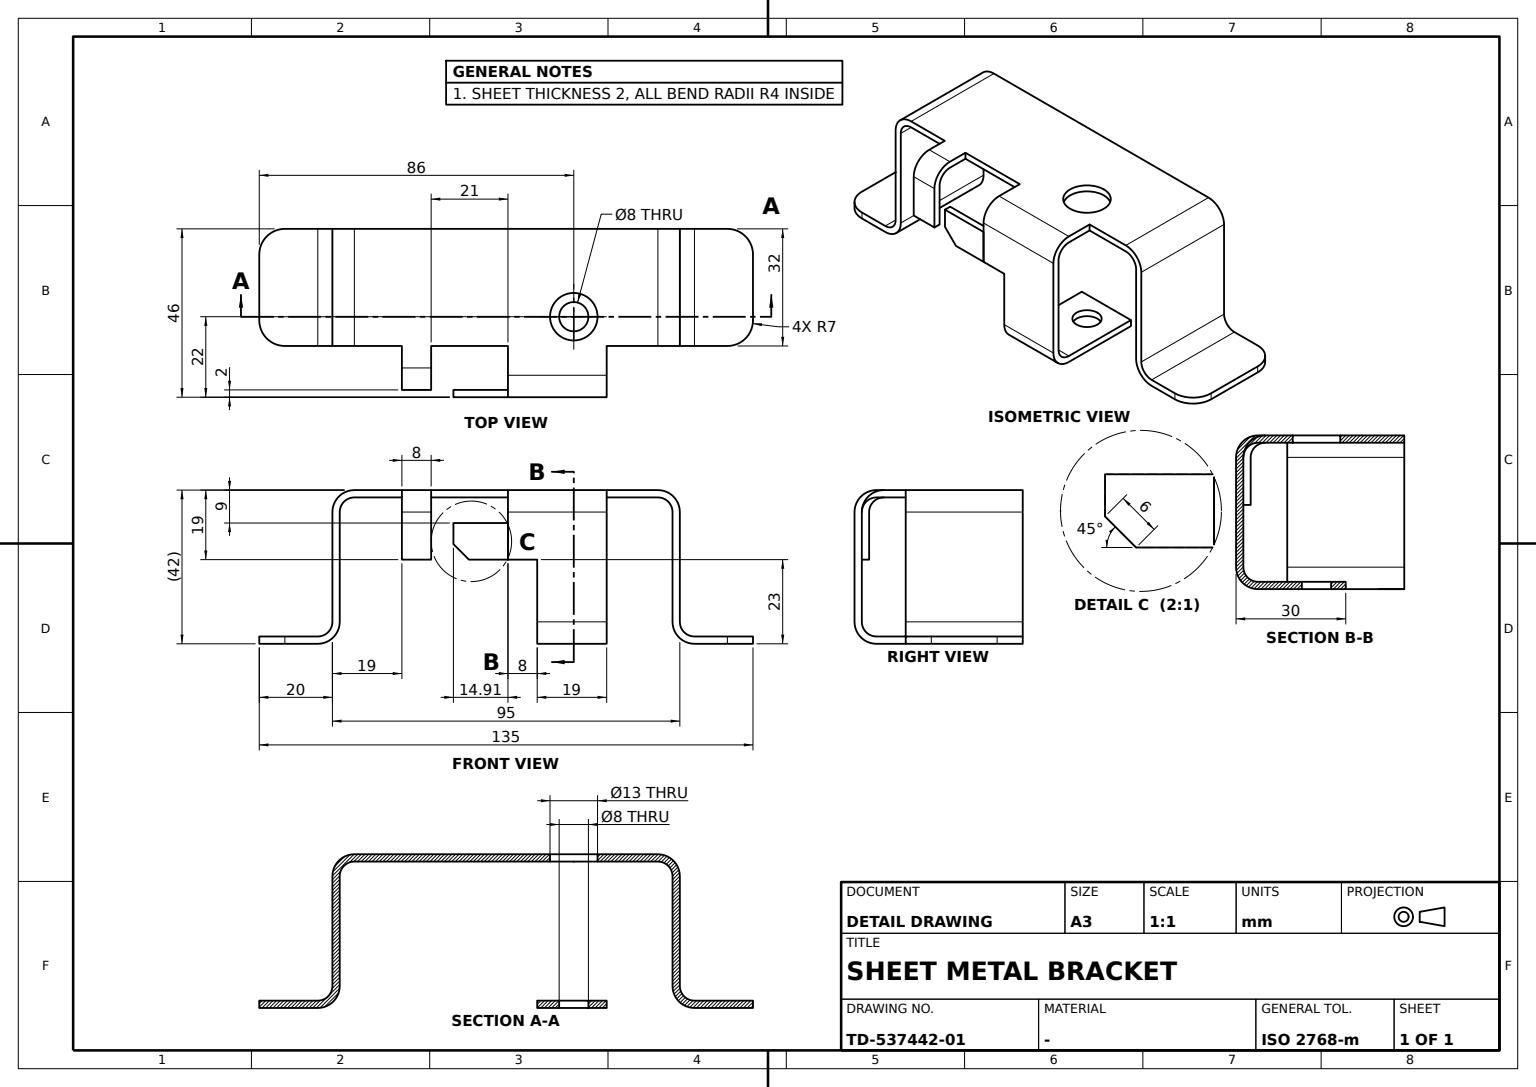
solid
v1 (0,27.5,-42)
v2 (0,27.5,-40)
e1 v1 v2 LINE
v3 (24,27.5,-40)
e2 v2 v3 LINE
v4 (28,27.5,-36)
e3 v3 v4 CIRCLE(AX(P(24,27.5,-36),D(0,1,0),D(0,0,1)),4) rev
v5 (28,27.5,-6)
e4 v5 v4 LINE
v6 (24,27.5,-2)
e5 v6 v5 CIRCLE(AX(P(24,27.5,-6),D(0,1,0),D(0,0,1)),4)
v7 (16,27.5,-2)
e6 v7 v6 LINE
v8 (16,27.5,0)
e7 v8 v7 LINE
v9 (24,27.5,0)
e8 v8 v9 LINE
v10 (30,27.5,-6)
e9 v9 v10 CIRCLE(AX(P(24,27.5,-6),D(0,1,0),D(0,0,1)),6)
v11 (30,27.5,-36)
e10 v11 v10 LINE
v12 (24,27.5,-42)
e11 v12 v11 CIRCLE(AX(P(24,27.5,-36),D(0,1,0),D(0,0,1)),6) rev
e12 v1 v12 LINE
face PLANE(AX(P(12,27.5,-42),D(0,1,0),D(1,0,0))) [e1 e2 e3 -e4 -e5 -e6 -e7 e8 e9 -e10 -e11 -e12]
v13 (24,0.5,-2)
e13 v6 v13 LINE
v14 (16,0.5,-2)
e14 v14 v13 LINE
v15 (16,-20.5,-2)
e15 v14 v15 LINE
v16 (22,-20.5,-2)
e16 v15 v16 LINE
v17 (22,-28.5,-2)
e17 v17 v16 LINE
v18 (16,-28.5,-2)
e18 v18 v17 LINE
v19 (16,-41.5,-2)
e19 v18 v19 LINE
v20 (-16,-41.5,-2)
e20 v19 v20 LINE
v21 (-16,41.5,-2)
e21 v20 v21 LINE
v22 (16,41.5,-2)
e22 v21 v22 LINE
e23 v22 v7 LINE
v23 (1.5,18.5,-2)
e24 v23 v23 CIRCLE(AX(P(8,18.5,-2),D(0,0,-1),D(-1,0,0)),6.5)
face PLANE(AX(P(16,0.5,-2),D(0,0,-1),D(0,1,0))) [e13 -e14 e15 e16 -e17 -e18 e19 e20 e21 e22 e23 e6] [-e24]
v24 (30,0.5,-6)
e25 v10 v24 LINE
v25 (30,0.5,-19)
e26 v25 v24 LINE
v26 (30,8.5,-19)
e27 v26 v25 LINE
v27 (30,8.5,-36)
e28 v26 v27 LINE
e29 v11 v27 LINE
face PLANE(AX(P(30,10.5,-2),D(1,0,0),D(0,-1,0))) [e25 -e26 -e27 e28 -e29 e10]
v28 (0,8.5,-42)
v29 (0,8.5,-40)
e30 v28 v29 LINE
e31 v29 v2 LINE
e32 v28 v1 LINE
face PLANE(AX(P(0,18,-42),D(1,0,0),D(0,0,1))) rev [e30 e31 -e1 -e32]
v30 (16,51.5,-40)
v31 (16,60.5,-40)
e33 v30 v31 LINE
v32 (16,47.5,-36)
e34 v30 v32 CIRCLE(AX(P(16,51.5,-36),D(-1,0,0),D(0,0,1)),4)
v33 (16,47.5,-6)
e35 v32 v33 LINE
v34 (16,41.5,0)
e36 v33 v34 CIRCLE(AX(P(16,41.5,-6),D(-1,0,0),D(0,0,1)),6) rev
e37 v34 v8 LINE
v35 (16,45.5,-6)
e38 v35 v22 CIRCLE(AX(P(16,41.5,-6),D(-1,0,0),D(0,0,1)),4) rev
v36 (16,45.5,-36)
e39 v35 v36 LINE
v37 (16,51.5,-42)
e40 v37 v36 CIRCLE(AX(P(16,51.5,-36),D(-1,0,0),D(0,0,1)),6)
v38 (16,60.5,-42)
e41 v37 v38 LINE
e42 v31 v38 LINE
face PLANE(AX(P(16,-47.5,0),D(-1,0,0),D(0,1,0))) rev [-e33 e34 e35 e36 e37 e7 -e23 -e38 e39 -e40 e41 -e42]
v39 (16,-47.5,-6)
v40 (16,-41.5,0)
e43 v39 v40 CIRCLE(AX(P(16,-41.5,-6),D(-1,0,0),D(0,0,1)),6)
v41 (-16,-41.5,0)
e44 v40 v41 LINE
v42 (-16,-47.5,-6)
e45 v42 v41 CIRCLE(AX(P(-16,-41.5,-6),D(-1,0,0),D(0,0,1)),6)
e46 v39 v42 LINE
face CYL(AX(P(0,-41.5,-6),D(-1,0,0),D(0,0,1)),6) [e43 e44 -e45 -e46]
v43 (-16,60.5,-42)
v44 (-9,67.5,-42)
e47 v43 v44 CIRCLE(AX(P(-9,60.5,-42),D(0,0,-1),D(-1,0,0)),7)
v45 (-16,60.5,-40)
e48 v45 v43 LINE
v46 (-9,67.5,-40)
e49 v45 v46 CIRCLE(AX(P(-9,60.5,-40),D(0,0,-1),D(-1,0,0)),7)
e50 v46 v44 LINE
face CYL(AX(P(-9,60.5,-40),D(0,0,-1),D(-1,0,0)),7) [-e47 -e48 e49 e50]
v47 (9,67.5,-40)
e51 v46 v47 LINE
v48 (-16,51.5,-40)
e52 v45 v48 LINE
e53 v30 v48 LINE
e54 v47 v31 CIRCLE(AX(P(9,60.5,-40),D(0,0,-1),D(-1,0,0)),7)
face PLANE(AX(P(28,18,-40),D(0,0,-1),D(0,-1,0))) rev [-e51 -e49 e52 -e53 e33 -e54]
v49 (-16,41.5,0)
e55 v41 v49 LINE
v50 (-16,47.5,-6)
e56 v50 v49 CIRCLE(AX(P(-16,41.5,-6),D(-1,0,0),D(0,0,1)),6) rev
v51 (-16,47.5,-36)
e57 v51 v50 LINE
e58 v48 v51 CIRCLE(AX(P(-16,51.5,-36),D(-1,0,0),D(0,0,1)),4)
v52 (-16,51.5,-42)
e59 v43 v52 LINE
v53 (-16,45.5,-36)
e60 v52 v53 CIRCLE(AX(P(-16,51.5,-36),D(-1,0,0),D(0,0,1)),6)
v54 (-16,45.5,-6)
e61 v54 v53 LINE
e62 v54 v21 CIRCLE(AX(P(-16,41.5,-6),D(-1,0,0),D(0,0,1)),4) rev
v55 (-16,-45.5,-6)
e63 v55 v20 CIRCLE(AX(P(-16,-41.5,-6),D(-1,0,0),D(0,0,1)),4)
v56 (-16,-45.5,-36)
e64 v55 v56 LINE
v57 (-16,-51.5,-42)
e65 v57 v56 CIRCLE(AX(P(-16,-51.5,-36),D(-1,0,0),D(0,0,1)),6) rev
v58 (-16,-60.5,-42)
e66 v57 v58 LINE
v59 (-16,-60.5,-40)
e67 v59 v58 LINE
v60 (-16,-51.5,-40)
e68 v60 v59 LINE
v61 (-16,-47.5,-36)
e69 v60 v61 CIRCLE(AX(P(-16,-51.5,-36),D(-1,0,0),D(0,0,1)),4) rev
e70 v61 v42 LINE
face PLANE(AX(P(-16,-59.5,-42),D(-1,0,0),D(0,1,0))) [e45 e55 -e56 -e57 -e58 -e52 e48 e59 e60 -e61 e62 -e21 -e63 e64 -e65 e66 -e67 -e68 e69 e70]
v62 (16,-45.5,-6)
e71 v62 v55 LINE
e72 v62 v19 CIRCLE(AX(P(16,-41.5,-6),D(-1,0,0),D(0,0,1)),4)
face CYL(AX(P(0,-41.5,-6),D(-1,0,0),D(0,0,1)),4) rev [e71 e63 -e20 -e72]
v63 (24,8.5,-42)
e73 v63 v27 CIRCLE(AX(P(24,8.5,-36),D(0,1,0),D(0,0,1)),6) rev
e74 v12 v63 LINE
face CYL(AX(P(24,14,-36),D(0,-1,0),D(1,0,0)),6) [e11 e29 -e73 -e74]
v64 (26,-28.5,-6)
v65 (26,-28.5,-19)
e75 v64 v65 LINE
v66 (26,-20.5,-6)
e76 v64 v66 LINE
v67 (26,-20.5,-19)
e77 v67 v66 LINE
e78 v65 v67 LINE
face PLANE(AX(P(26,0,-2),D(1,0,0),D(0,-1,0))) rev [-e75 e76 -e77 -e78]
v68 (16,-47.5,-36)
e79 v61 v68 LINE
e80 v68 v39 LINE
face PLANE(AX(P(0,-47.5,-2),D(0,-1,0),D(-1,0,0))) [e79 e80 e46 -e70]
v69 (4,18.5,-42)
e81 v69 v69 CIRCLE(AX(P(8,18.5,-42),D(0,0,-1),D(-1,0,0)),4)
v70 (4,18.5,-40)
e82 v70 v70 CIRCLE(AX(P(8,18.5,-40),D(0,0,-1),D(-1,0,0)),4)
face CYL(AX(P(8,18.5,-41),D(0,0,-1),D(1,0,0)),4) rev [e81] [-e82]
v71 (9,67.5,-42)
e83 v71 v38 CIRCLE(AX(P(9,60.5,-42),D(0,0,-1),D(-1,0,0)),7)
e84 v47 v71 LINE
face CYL(AX(P(9,60.5,-40),D(0,0,-1),D(-1,0,0)),7) [e54 e42 -e83 -e84]
e85 v36 v53 LINE
e86 v37 v52 LINE
face CYL(AX(P(0,51.5,-36),D(-1,0,0),D(0,-1,0)),6) [e40 e85 -e60 -e86]
v72 (16,-51.5,-42)
e87 v57 v72 LINE
v73 (16,-45.5,-36)
e88 v56 v73 LINE
e89 v72 v73 CIRCLE(AX(P(16,-51.5,-36),D(-1,0,0),D(0,0,1)),6) rev
face CYL(AX(P(0,-51.5,-36),D(1,0,0),D(0,1,0)),6) [-e87 e65 e88 -e89]
v74 (1.5,18.5,0)
e90 v74 v74 CIRCLE(AX(P(8,18.5,0),D(0,0,-1),D(-1,0,0)),6.5) rev
face CYL(AX(P(8,18.5,-1),D(0,0,-1),D(1,0,0)),6.5) rev [e24] [e90]
v75 (16,0.5,0)
e91 v75 v14 LINE
v76 (16,-20.5,0)
e92 v75 v76 LINE
e93 v76 v15 LINE
face PLANE(AX(P(16,-47.5,0),D(-1,0,0),D(0,1,0))) rev [-e91 e92 e93 -e15]
e94 v71 v44 LINE
face PLANE(AX(P(28,18,-42),D(0,0,-1),D(0,-1,0))) [e47 -e94 e83 -e41 e86 -e59]
v77 (-9,-67.5,-40)
e95 v77 v59 CIRCLE(AX(P(-9,-60.5,-40),D(0,0,-1),D(-1,0,0)),7)
v78 (-9,-67.5,-42)
e96 v78 v58 CIRCLE(AX(P(-9,-60.5,-42),D(0,0,-1),D(-1,0,0)),7)
e97 v77 v78 LINE
face CYL(AX(P(-9,-60.5,-40),D(0,0,-1),D(1,0,0)),7) [e95 e67 -e96 -e97]
e98 v16 v66 CIRCLE(AX(P(22,-20.5,-6),D(0,1,0),D(0,0,1)),4)
v79 (22,-20.5,0)
e99 v76 v79 LINE
v80 (28,-20.5,-6)
e100 v79 v80 CIRCLE(AX(P(22,-20.5,-6),D(0,1,0),D(0,0,1)),6)
v81 (28,-20.5,-19)
e101 v81 v80 LINE
e102 v81 v67 LINE
face PLANE(AX(P(28,-20.5,-12.5),D(0,1,0),D(1,0,0))) [e77 -e98 -e16 -e93 e99 e100 -e101 e102]
e103 v17 v64 CIRCLE(AX(P(22,-28.5,-6),D(0,1,0),D(0,0,1)),4)
face CYL(AX(P(22,-24.5,-6),D(0,1,0),D(0,0,1)),4) rev [e17 e98 -e76 -e103]
e104 v32 v51 LINE
e105 v50 v33 LINE
face PLANE(AX(P(0,47.5,-2),D(0,1,0),D(1,0,0))) [e104 e57 e105 -e35]
v82 (16,-60.5,-42)
e106 v82 v72 LINE
v83 (9,-67.5,-42)
e107 v82 v83 CIRCLE(AX(P(9,-60.5,-42),D(0,0,-1),D(-1,0,0)),7)
e108 v78 v83 LINE
face PLANE(AX(P(28,18,-42),D(0,0,-1),D(0,-1,0))) [-e66 e87 -e106 e107 -e108 e96]
face PLANE(AX(P(0,67.5,-42),D(0,-1,0),D(1,0,0))) rev [-e50 e51 e84 e94]
v84 (22,-28.5,0)
e109 v84 v79 LINE
v85 (24,0.5,0)
e110 v75 v85 LINE
e111 v9 v85 LINE
e112 v49 v34 LINE
v86 (16,-28.5,0)
e113 v86 v40 LINE
e114 v86 v84 LINE
face PLANE(AX(P(16,0.5,0),D(0,0,-1),D(0,1,0))) rev [e109 -e99 -e92 e110 -e111 -e8 -e37 -e112 -e55 -e44 -e113 e114] [-e90]
v87 (28,-28.5,-6)
e115 v84 v87 CIRCLE(AX(P(22,-28.5,-6),D(0,1,0),D(0,0,1)),6)
e116 v86 v18 LINE
v88 (28,-28.5,-19)
e117 v88 v65 LINE
e118 v87 v88 LINE
face PLANE(AX(P(22,-28.5,0),D(0,1,0),D(0.923879533,0,-0.382683432))) rev [-e115 -e114 e116 e18 e103 e75 -e117 -e118]
v89 (9,-67.5,-40)
e119 v89 v77 LINE
v90 (16,-60.5,-40)
e120 v90 v89 CIRCLE(AX(P(9,-60.5,-40),D(0,0,-1),D(-1,0,0)),7)
v91 (16,-51.5,-40)
e121 v90 v91 LINE
e122 v60 v91 LINE
face PLANE(AX(P(28,18,-40),D(0,0,-1),D(0,-1,0))) rev [-e119 -e120 e121 -e122 e68 -e95]
e123 v54 v35 LINE
face CYL(AX(P(0,41.5,-6),D(1,0,0),D(0,0,1)),4) rev [e123 e38 -e22 -e62]
e124 v87 v80 LINE
face CYL(AX(P(22,-24.5,-6),D(0,1,0),D(0,0,1)),6) [-e100 -e109 e115 e124]
v92 (24,8.5,-40)
e125 v92 v29 LINE
e126 v3 v92 LINE
face PLANE(AX(P(28,18,-40),D(0,0,-1),D(0,-1,0))) rev [e82] [-e31 -e125 -e126 -e2]
face CYL(AX(P(0,41.5,-6),D(1,0,0),D(0,0,1)),6) [e112 -e36 -e105 e56]
e127 v91 v68 CIRCLE(AX(P(16,-51.5,-36),D(-1,0,0),D(0,0,1)),4) rev
face CYL(AX(P(0,-51.5,-36),D(1,0,0),D(0,1,0)),4) rev [-e69 e122 e127 -e79]
v93 (28,0.5,-19)
e128 v25 v93 LINE
v94 (28,8.5,-19)
e129 v94 v93 LINE
e130 v26 v94 LINE
face PLANE(AX(P(30,4.5,-19),D(0,0,1),D(1,0,0))) rev [e128 -e129 -e130 e27]
e131 v90 v82 LINE
e132 v62 v73 LINE
face PLANE(AX(P(16,-47.5,0),D(-1,0,0),D(0,1,0))) rev [e113 -e43 -e80 -e127 -e121 e131 e106 e89 -e132 e72 -e19 -e116]
e133 v85 v24 CIRCLE(AX(P(24,0.5,-6),D(0,1,0),D(0,0,1)),6)
face CYL(AX(P(24,14,-6),D(0,-1,0),D(0,0,1)),6) [-e9 e111 e133 -e25]
e134 v89 v83 LINE
face PLANE(AX(P(0,-67.5,-42),D(0,1,0),D(1,0,0))) rev [e108 -e134 e119 e97]
v95 (28,8.5,-36)
e135 v94 v95 LINE
e136 v92 v95 CIRCLE(AX(P(24,8.5,-36),D(0,1,0),D(0,0,1)),4) rev
e137 v63 v28 LINE
face PLANE(AX(P(12,8.5,-42),D(0,1,0),D(1,0,0))) rev [e73 -e28 e130 e135 -e136 e125 -e30 -e137]
face PLANE(AX(P(28,18,-42),D(0,0,-1),D(0,-1,0))) [-e81] [e74 e137 e32 e12]
e138 v88 v81 LINE
face PLANE(AX(P(30,4.5,-19),D(0,0,1),D(1,0,0))) rev [-e102 -e138 e117 e78]
e139 v4 v95 LINE
face CYL(AX(P(24,14,-36),D(0,-1,0),D(1,0,0)),4) rev [-e3 e126 e136 -e139]
face CYL(AX(P(9,-60.5,-40),D(0,0,-1),D(1,0,0)),7) [e120 e134 -e107 -e131]
v96 (28,0.5,-6)
e140 v96 v93 LINE
e141 v5 v96 LINE
face PLANE(AX(P(28,10.5,-2),D(1,0,0),D(0,-1,0))) rev [e139 -e135 e129 -e140 -e141 e4]
face PLANE(AX(P(0,45.5,-2),D(0,1,0),D(1,0,0))) rev [-e123 e61 -e85 -e39]
e142 v13 v96 CIRCLE(AX(P(24,0.5,-6),D(0,1,0),D(0,0,1)),4)
face PLANE(AX(P(30,0.5,-24),D(0,1,0),D(1,0,0))) rev [e26 -e133 -e110 e91 e14 e142 e140 -e128]
face CYL(AX(P(24,14,-6),D(0,-1,0),D(0,0,1)),4) rev [e141 -e142 -e13 e5]
face PLANE(AX(P(28,10.5,-2),D(1,0,0),D(0,-1,0))) [-e124 e118 e138 e101]
face PLANE(AX(P(0,-45.5,-2),D(0,-1,0),D(-1,0,0))) rev [-e88 -e64 -e71 e132]
face CYL(AX(P(0,51.5,-36),D(-1,0,0),D(0,-1,0)),4) rev [-e104 -e34 e53 e58]
solid
v97 (28,0.5,-19)
v98 (30,0.5,-19)
e143 v97 v98 LINE
v99 (28,0.5,-9)
e144 v97 v99 LINE
v100 (30,0.5,-9)
e145 v99 v100 LINE
e146 v98 v100 LINE
face PLANE(AX(P(30,0.5,-19),D(0,-1,0),D(0,0,1))) rev [-e143 e144 e145 -e146]
v101 (28,-10.17,-19)
e147 v97 v101 LINE
v102 (28,-14.412641,-14.757359)
e148 v102 v101 LINE
v103 (28,-14.412641,-9)
e149 v103 v102 LINE
e150 v103 v99 LINE
face PLANE(AX(P(28,0,0),D(1,0,0),D(0,1,0))) rev [-e144 e147 -e148 -e149 e150]
v104 (30,-14.412641,-14.757359)
e151 v102 v104 LINE
v105 (30,-14.412641,-9)
e152 v105 v104 LINE
e153 v103 v105 LINE
face PLANE(AX(P(30,-14.412641,-9),D(0,1,0),D(0,0,-1))) rev [e149 e151 -e152 -e153]
e154 v105 v100 LINE
face PLANE(AX(P(30,0.5,-9),D(0,0,-1),D(0,-1,0))) rev [-e145 -e150 e153 e154]
v106 (30,-10.17,-19)
e155 v104 v106 LINE
e156 v98 v106 LINE
face PLANE(AX(P(30,0,0),D(1,0,0),D(0,1,0))) [e152 e155 -e156 e146 -e154]
e157 v101 v106 LINE
face PLANE(AX(P(30,-10.17,-19),D(0,0,1),D(0,1,0))) rev [e143 e156 -e157 -e147]
face PLANE(AX(P(30,-14.412641,-14.757359),D(0,0.707106781,0.707106781),D(0,0.707106781,-0.707106781))) rev [e157 -e155 -e151 e148]
